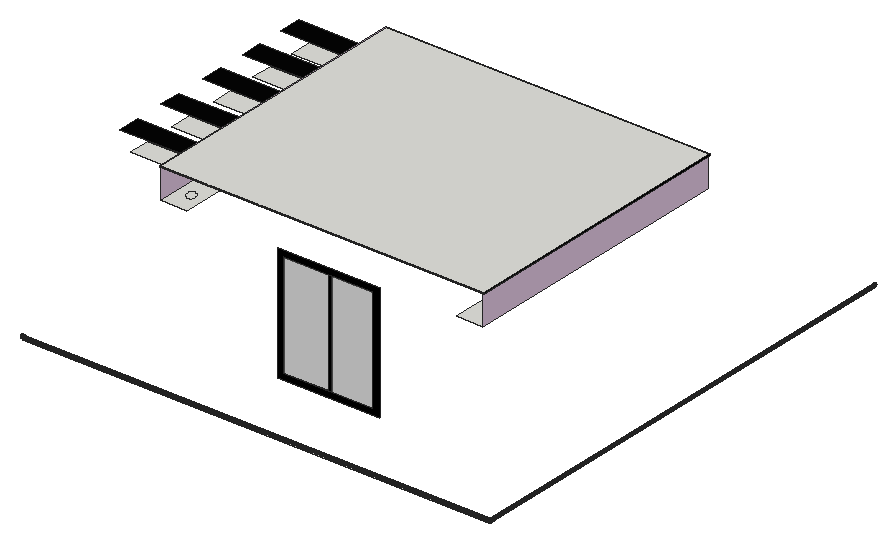
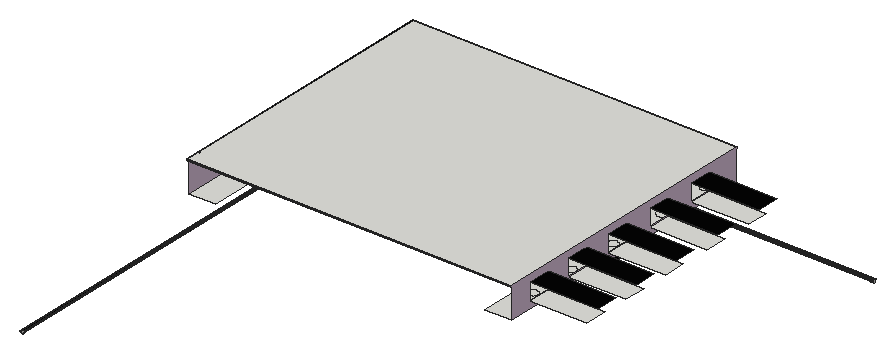
# SketchUp Ruby script. Lengths in inches.
U = 1.inch
M = Sketchup.active_model
def pt(a) = Geom::Point3d.new(a.map { |v| v * U })
def face(e, loops, mat)
  f = e.add_face(loops[0].map { |a| pt(a) })
  loops[1..].each { |l| e.add_face(l.map { |a| pt(a) }).erase! }
  f.material = f.back_material = mat if mat
  f
end
# faces: each face lists its corners as indices into pts; further lists are holes
def faces(e, pts, list, mat = nil) = list.each { |f| face(e, (f[0].is_a?(Array) ? f : [f]).map { |l| l.map { |i| pts[i] } }, mat) }
# xy, xz, yz: faces in a plane at the given z, y or x. An outline is a flat list of corners, or four numbers for a rectangle; further outlines are holes
def ring(l) = l.size == 4 ? [[l[0], l[1]], [l[2], l[1]], [l[2], l[3]], [l[0], l[3]]] : l.each_slice(2).to_a
def flat(e, list, mat, &to3) = list.each { |f| face(e, (f[0].is_a?(Array) ? f : [f]).map { |l| ring(l).map { |u, v| to3.(u, v) } }, mat) }
def xy(e, z, list, mat = nil) = flat(e, list, mat) { |x, y| [x, y, z] }
def xz(e, y, list, mat = nil) = flat(e, list, mat) { |x, z| [x, y, z] }
def yz(e, x, list, mat = nil) = flat(e, list, mat) { |y, z| [x, y, z] }
def lines(e, pts, list) = list.each { |a, b| e.add_line(pt(pts[a]), pt(pts[b])) }
# prism: a flat outline (further loops are holes) pulled along v
def prism(e, loops, v, mat = nil)
  f = face(e, loops, mat); d = Geom::Vector3d.new(v.map { |x| x * U })
  f.pushpull(f.normal.samedirection?(d) ? d.length : -d.length)
end
def box(e, o, s, mat = nil) = prism(e, [[o, [o[0] + s[0], o[1], o[2]], [o[0] + s[0], o[1] + s[1], o[2]], [o[0], o[1] + s[1], o[2]]]], [0, 0, s[2]], mat)
def at(x, y, z, deg = 0) = Geom::Transformation.translation(pt([x, y, z])) * Geom::Transformation.rotation(ORIGIN, Z_AXIS, deg.degrees)
def axes(o, x, y, z) = Geom::Transformation.new([*x, 0, *y, 0, *z, 0, *pt(o).to_a, 1])
def part(name) = M.definitions.add(name)
# library, detail: a bought-in or finely detailed component or shape, given as its bounding box
def library(name, o, s) = part(name).tap { |d| box(d.entities, o, s) }
def detail(e, o, s) = box(e.add_group.entities, o, s)
def put(e, d, t, mat = nil) = e.add_instance(d, t).tap { |i| i.material = mat if mat }
def group(e, t, mat = nil) = e.add_group.tap { |g| g.transformation = t; g.material = mat if mat }.entities
root = M.entities
M.materials.add("[0118_Thistle]").color = [216, 191, 216]
M.materials.add("[0136_Charcoal]").color = [5, 5, 5]
M.materials.add("[0137_Black]").color = [0, 0, 0]
M.materials.add("[Translucent Glass Gray]").color = [128, 128, 128]
M.materials["[Translucent Glass Gray]"].alpha = 0.5
xy(root,1352.375,[[8.99,75.58,1077.01,78.58]])
xy(root,1354.0625,[[1079.8,75.38,1080.11,75.38,1080.42,75.4,1080.73,75.47,1081.03,75.56,1081.32,75.68,1081.59,75.83,1081.85,76.01,1082.09,76.22,1082.3,76.45,1082.49,76.7,1082.65,76.97,1082.78,77.26,1082.89,77.55,1082.96,77.86,1082.99,78.17,1083,78.48,1082.97,78.8,1082.91,79.11,1082.82,79.41,1082.69,79.69,1082.54,79.97,1082.36,80.23,1082.15,80.46,1081.92,80.68,1081.67,80.86,1081.4,81.03,1081.12,81.16,1080.82,81.26,1080.52,81.33,1080.2,81.37,1079.89,81.37,1079.58,81.35,1079.27,81.28,1078.97,81.19,1078.68,81.07,1078.41,80.92,1078.15,80.74,1077.91,80.53,1077.7,80.3,1077.51,80.05,1077.35,79.78,1077.22,79.49,1077.11,79.2,1077.04,78.89,1077.01,78.58,1077,78.375,1077,78.27,1077.03,77.95,1077.09,77.64,1077.18,77.34,1077.31,77.06,1077.46,76.78,1077.64,76.52,1077.85,76.29,1078.08,76.07,1078.33,75.89,1078.6,75.72,1078.88,75.59,1079.18,75.49,1079.48,75.42]])
xy(root,1354.07,[[1079.86,81.375,1080.18,1173.38]],"[0137_Black]")
xy(root,1360.06,[[1079.82,81.375,1080.14,1179.37]],"[0137_Black]")
xy(root,1597.0625,[[[156,288.375,216,930.375],[186.49,446.54,189.62,446.78,192.57,447.82,195.16,449.58,197.2,451.96,198.55,454.78,199.13,457.86,198.9,460.99,197.86,463.94,196.09,466.53,193.72,468.57,190.89,469.93,187.8125,470.5,184.6875,470.27,181.73,469.23,179.15,467.46,177.11,465.09,175.75,462.26,175.17,459.18,175.41,456.06,176.45,453.1,178.21,450.52,180.59,448.48,183.41,447.12],[186.49,587.35,189.62,587.59,192.57,588.63,195.16,590.4,197.2,592.77,198.55,595.6,199.13,598.68,198.9,601.8,197.86,604.75,196.09,607.34,193.72,609.38,190.89,610.74,187.8125,611.32,184.6875,611.08,181.73,610.04,179.15,608.28,177.11,605.9,175.75,603.07,175.17,600,175.41,596.87,176.45,593.92,178.21,591.33,180.59,589.29,183.41,587.93],[186.49,708.35,189.62,708.59,192.57,709.63,195.16,711.4,197.2,713.77,198.55,716.6,199.13,719.68,198.9,722.8,197.86,725.75,196.09,728.34,193.72,730.38,190.89,731.74,187.8125,732.32,184.6875,732.08,181.73,731.04,179.15,729.28,177.11,726.9,175.75,724.07,175.17,721,175.41,717.87,176.45,714.92,178.21,712.33,180.59,710.29,183.41,708.93],[186.49,324.85,189.62,325.09,192.57,326.13,195.16,327.9,197.2,330.27,198.55,333.1,199.13,336.18,198.9,339.3,197.86,342.25,196.09,344.84,193.72,346.88,190.89,348.24,187.8125,348.82,184.6875,348.58,181.73,347.54,179.15,345.78,177.11,343.4,175.75,340.57,175.17,337.5,175.41,334.37,176.45,331.42,178.21,328.83,180.59,326.79,183.41,325.43],[186.49,817.29,189.62,817.53,192.57,818.57,195.16,820.33,197.2,822.71,198.55,825.53,199.13,828.61,198.9,831.74,197.86,834.69,196.09,837.28,193.72,839.32,190.89,840.68,187.8125,841.25,184.6875,841.02,181.73,839.98,179.15,838.21,177.11,835.84,175.75,833.01,175.17,829.93,175.41,826.81,176.45,823.85,178.21,821.27,180.59,819.23,183.41,817.87]],[834,288.375,894,930.375],[186.49,324.85,183.41,325.43,180.59,326.79,178.21,328.83,176.45,331.42,175.41,334.37,175.17,337.5,175.75,340.57,177.11,343.4,179.15,345.78,181.73,347.54,184.6875,348.58,187.8125,348.82,190.89,348.24,193.72,346.88,196.09,344.84,197.86,342.25,198.9,339.3,199.13,336.18,198.55,333.1,197.2,330.27,195.16,327.9,192.57,326.13,189.62,325.09],[186.49,446.54,183.41,447.12,180.59,448.48,178.21,450.52,176.45,453.1,175.41,456.06,175.17,459.18,175.75,462.26,177.11,465.09,179.15,467.46,181.73,469.23,184.6875,470.27,187.8125,470.5,190.89,469.93,193.72,468.57,196.09,466.53,197.86,463.94,198.9,460.99,199.13,457.86,198.55,454.78,197.2,451.96,195.16,449.58,192.57,447.82,189.62,446.78],[186.49,587.35,183.41,587.93,180.59,589.29,178.21,591.33,176.45,593.92,175.41,596.87,175.17,600,175.75,603.07,177.11,605.9,179.15,608.28,181.73,610.04,184.6875,611.08,187.8125,611.32,190.89,610.74,193.72,609.38,196.09,607.34,197.86,604.75,198.9,601.8,199.13,598.68,198.55,595.6,197.2,592.77,195.16,590.4,192.57,588.63,189.62,587.59],
  [186.49,708.35,183.41,708.93,180.59,710.29,178.21,712.33,176.45,714.92,175.41,717.87,175.17,721,175.75,724.07,177.11,726.9,179.15,729.28,181.73,731.04,184.6875,732.08,187.8125,732.32,190.89,731.74,193.72,730.38,196.09,728.34,197.86,725.75,198.9,722.8,199.13,719.68,198.55,716.6,197.2,713.77,195.16,711.4,192.57,709.63,189.62,708.59],[186.49,817.29,183.41,817.87,180.59,819.23,178.21,821.27,176.45,823.85,175.41,826.81,175.17,829.93,175.75,833.01,177.11,835.84,179.15,838.21,181.73,839.98,184.6875,841.02,187.8125,841.25,190.89,840.68,193.72,839.32,196.09,837.28,197.86,834.69,198.9,831.74,199.13,828.61,198.55,825.53,197.2,822.71,195.16,820.33,192.57,818.57,189.62,817.53]])
xy(root,1614.61,[[24.25,366.56,156,417.12],[24.25,484.62,156,535.18],[24.25,604.12,156,654.68],[24.25,717.12,156,767.68],[24.25,827.68,156,878.24]])
xy(root,1652.92,[[0,366.56,156,417.12],[0,484.62,156,535.18],[0,604.12,156,654.68],[0,717.12,156,767.68],[0,827.68,156,878.24]],"[0136_Charcoal]")
xy(root,1666.0625,[[156,285.375,897,288.375],[894,288.375,897,933.375],[156,930.375,894,933.375]])
xy(root,1669.0625,[[156,285.375,897,933.375]])
xz(root,81.375,[[5.97,1354.0625,6,1354.0625,6,1357.0625,9,1357.0625,8.99,1357.35,8.94,1357.66,8.86,1357.97,8.75,1358.26,8.61,1358.54,8.44,1358.81,8.25,1359.05,8.03,1359.28,7.78,1359.47,7.52,1359.65,7.24,1359.79,6.95,1359.91,6.65,1359.99,6.34,1360.04,6.03,1360.0625,5.71,1360.05,5.4,1360,5.1,1359.92,4.8,1359.8125,4.52,1359.67,4.26,1359.5,4.01,1359.31,3.79,1359.09,3.59,1358.85,3.41,1358.58,3.27,1358.31,3.15,1358.01,3.07,1357.71,3.02,1357.4,3,1357.09,3.01,1356.77,3.06,1356.46,3.14,1356.16,3.25,1355.87,3.39,1355.58,3.56,1355.32,3.75,1355.07,3.97,1354.85,4.22,1354.65,4.48,1354.48,4.76,1354.33,5.05,1354.22,5.35,1354.13,5.66,1354.08],[6,1354.0625,6.29,1354.08,6.6,1354.12,6.9,1354.2,7.2,1354.3125,7.48,1354.45,7.74,1354.62,7.99,1354.82,8.21,1355.04,8.41,1355.28,8.59,1355.54,8.73,1355.82,8.85,1356.11,8.93,1356.41,8.98,1356.72,9,1357.04,9,1357.0625,6,1357.0625],[1079.86,1354.07,1080.18,1354.07,1080.49,1354.1,1080.79,1354.17,1081.09,1354.27,1081.38,1354.4,1081.65,1354.56,1081.9,1354.74,1082.13,1354.95,1082.34,1355.1875,1082.53,1355.44,1082.68,1355.72,1082.81,1356,1082.9,1356.3,1082.97,1356.61,1083,1356.92,1082.99,1357.24,1082.96,1357.55,1082.89,1357.86,1082.79,1358.15,1082.66,1358.44,1082.51,1358.71,1082.32,1358.96,1082.11,1359.2,1081.875,1359.41,1081.62,1359.59,1081.35,1359.74,1081.06,1359.87,1080.76,1359.96,1080.45,1360.03,1080.14,1360.06,1079.82,1360.06,1079.51,1360.02,1079.21,1359.96,1078.91,1359.86,1078.62,1359.73,1078.35,1359.57,1078.1,1359.38,1077.87,1359.17,1077.66,1358.9375,1077.47,1358.68,1077.32,1358.41,1077.19,1358.12,1077.1,1357.82,1077.03,1357.51,1077,1357.2,1077,1357.0625,1077.01,1356.89,1077.04,1356.57,1077.11,1356.27,1077.21,1355.97,1077.34,1355.68,1077.49,1355.41,1077.68,1355.16,1077.89,1354.93,1078.125,1354.72,1078.38,1354.54,1078.65,1354.38,1078.94,1354.26,1079.24,1354.16,1079.55,1354.1]])
xz(root,285.375,[[156,1666.0625,897,1669.0625]],"[0137_Black]")
xz(root,288.375,[[[423.26,1325.51,656.88,1594.07],[437.95,1340.2,642.2,1579.38]],[540.07,1340.2,547.42,1579.38]],"[0137_Black]")
xz(root,288.375,[[437.95,1340.2,540.07,1579.38],[547.42,1340.2,642.2,1579.38]],"[Translucent Glass Gray]")
xz(root,933.375,[[156,1666.0625,897,1669.0625]],"[0137_Black]")
yz(root,156,[[[288.375,1597.0625,288.375,1666.0625,285.375,1666.0625,285.375,1669.0625,933.375,1669.0625,933.375,1666.0625,930.375,1666.0625,930.375,1597.0625],[827.68,1614.61,878.24,1652.92],[717.12,1614.61,767.68,1652.92],[604.12,1614.61,654.68,1652.92],[484.62,1614.61,535.18,1652.92],[366.56,1614.61,417.12,1652.92]]],"[0118_Thistle]")
yz(root,894,[[288.375,1597.0625,930.375,1666.0625]],"[0118_Thistle]")
yz(root,897,[[285.375,1666.0625,933.375,1669.0625]],"[0137_Black]")
p = [[8.85,77.45,1354.21],[8.93,77.75,1354.13],[1080,77.75,1354.13],[1080,77.45,1354.21],[8.98,78.0625,1354.08],[1080,78.0625,1354.08],
  [9,78.375,1354.0625],[1077,78.375,1354.0625],[1080,78.375,1354.0625],[8.98,78.6875,1354.08],[1080,78.6875,1354.08],[8.93,79,1354.13],
  [1080,79,1354.13],[8.85,79.3,1354.21],[1080,79.3,1354.21],[1079.24,1173.47,1354.16],[1079.55,1173.41,1354.1],[1079.55,81.375,1354.1],
  [1079.24,81.375,1354.16],[1079.86,1173.38,1354.07],[1079.86,81.375,1354.07],[1080.18,1173.38,1354.07],[1080.49,1173.41,1354.1],[1080.49,81.375,1354.1],
  [1080.18,81.375,1354.07],[1080.79,1173.48,1354.17],[1080.79,81.375,1354.17],[1077.01,1176.2,1354.09],[1077.01,1175.79,1354.12],[1077.01,1175.05,1354.37],
  [1077.02,1174.4,1354.81],[1077.02,1173.88,1355.4],[1077.02,1173.53,1356.1],[1077.02,1173.38,1356.87],[1077.02,1173.43,1357.65],[1077.02,1173.69,1358.39],
  [1077.02,1174.12,1359.04],[1077.01,1174.71,1359.56],[1077.01,1175.41,1359.9],[1077.01,1176.18,1360.06],[1077,1176.96,1360],[1077,1177.7,1359.75],
  [1076.99,1178.35,1359.32],[1076.99,1178.87,1358.73],[1076.99,1179.22,1358.03],[1076.99,1179.37,1357.26],[1076.99,1179.32,1356.48],[1076.99,1179.06,1355.73],
  [1076.99,1178.63,1355.08],[1076.99,1178.04,1354.57],[1077,1177.34,1354.22],[1077,1176.57,1354.07],[1077,1176.51,1354.07],[1077,1176.51,1357.2],
  [1077,1176.375,1357.0625],[1077.01,1176.2,1356.89],[8.74,77.15,1354.32],[1080,77.15,1354.32],[8.74,79.6,1354.32],[1080,79.6,1354.32],
  [1078.94,1173.57,1354.26],[1078.94,81.375,1354.26],[1081.09,1173.58,1354.27],[1081.09,81.375,1354.27],[8.6,76.875,1354.46],[1080,76.875,1354.46],
  [8.6,79.875,1354.46],[1080,79.875,1354.46],[1078.65,1173.69,1354.38],[1078.65,81.375,1354.38],[1081.38,1173.71,1354.4],[1081.38,81.375,1354.4],
  [1078.38,1173.85,1354.54],[1078.38,81.375,1354.54],[1081.65,1173.87,1354.56],[1081.65,81.375,1354.56],[8.43,76.61,1354.64],[1080,76.61,1354.64],
  [8.43,80.14,1354.64],[1080,80.14,1354.64],[1078.125,1174.03,1354.72],[1078.125,81.375,1354.72],[8.23,76.37,1354.83],[1080,76.37,1354.83],
  [8.23,80.38,1354.83],[1080,80.38,1354.83],[1081.9,1174.06,1354.74],[1081.9,81.375,1354.74],[1077.89,1174.24,1354.93],[1077.89,81.375,1354.93],
  [1082.13,1174.27,1354.95],[1082.13,81.375,1354.95],[8.01,76.15,1355.06],[1080,76.15,1355.06],[8.01,80.6,1355.06],[1080,80.6,1355.06],
  [1077.68,1174.47,1355.16],[1077.68,81.375,1355.16],[1082.34,1174.5,1355.1875],[1082.34,81.375,1355.1875],[7.76,75.95,1355.3],[1080,75.95,1355.3],
  [7.76,80.8,1355.3],[1080,80.8,1355.3],[1077.49,1174.73,1355.41],[1077.49,81.375,1355.41],[1082.53,1174.76,1355.44],[1082.53,81.375,1355.44],
  [7.5,75.78,1355.5625],[1080,75.78,1355.5625],[7.5,80.97,1355.5625],[1080,80.97,1355.5625],[1077.34,1175,1355.68],[1077.34,81.375,1355.68],
  [1082.68,1175.03,1355.72],[1082.68,81.375,1355.72],[7.22,75.63,1355.84],[1080,75.63,1355.84],[7.22,81.12,1355.84],[1080,81.12,1355.84],
  [1077.21,1175.28,1355.97],[1077.21,81.375,1355.97],[1082.81,1175.32,1356],[1082.81,81.375,1356],[6.93,75.52,1356.14],[1080,75.52,1356.14],
  [6.93,81.23,1356.14],[1080,81.23,1356.14],[1077.11,1175.58,1356.27],[1077.11,81.375,1356.27],[1082.9,1175.62,1356.3],[1082.9,81.375,1356.3],
  [6.625,75.44,1356.4375],[1080,75.44,1356.4375],[6.625,81.31,1356.4375],[1080,81.31,1356.4375],[1077.04,1175.89,1356.57],[1077.04,81.375,1356.57],
  [1082.97,1175.92,1356.61],[1082.97,81.375,1356.61],[6.3125,75.39,1356.75],[1080,75.39,1356.75],[6.3125,81.36,1356.75],[1080,81.36,1356.75],
  [1077.01,81.375,1356.89],[1083,1176.24,1356.92],[1083,81.375,1356.92],[6,75.375,1357.0625],[1080,75.375,1357.0625],[6,81.375,1357.0625],
  [9,81.375,1357.0625],[1077,81.375,1357.0625],[1080,81.375,1357.0625],[1077,81.375,1357.2],[1082.99,1176.55,1357.24],[1082.99,81.375,1357.24],
  [5.6875,75.39,1357.375],[1080,75.39,1357.375],[5.6875,81.36,1357.375],[1080,81.36,1357.375],[1077.03,1176.83,1357.51],[1077.03,81.375,1357.51],
  [1082.96,1176.86,1357.55],[1082.96,81.375,1357.55],[5.375,75.44,1357.6875],[1080,75.44,1357.6875],[5.375,81.31,1357.6875],[1080,81.31,1357.6875],
  [1077.1,1177.13,1357.82],[1077.1,81.375,1357.82],[1082.89,1177.17,1357.86],[1082.89,81.375,1357.86],[5.07,75.52,1357.99],[1080,75.52,1357.99],
  [5.07,81.23,1357.99],[1080,81.23,1357.99],[1077.19,1177.43,1358.12],[1077.19,81.375,1358.12],[1082.79,1177.47,1358.15],[1082.79,81.375,1358.15],
  [4.78,75.63,1358.28],[1080,75.63,1358.28],[4.78,81.12,1358.28],[1080,81.12,1358.28],[1077.32,1177.72,1358.41],[1077.32,81.375,1358.41],
  [1082.66,1177.75,1358.44],[1082.66,81.375,1358.44],[4.5,75.78,1358.5625],[1080,75.78,1358.5625],[4.5,80.97,1358.5625],[1080,80.97,1358.5625],
  [1077.47,1177.99,1358.68],[1077.47,81.375,1358.68],[1082.51,1178.02,1358.71],[1082.51,81.375,1358.71],[4.24,75.95,1358.83],[1080,75.95,1358.83],
  [4.24,80.8,1358.83],[1080,80.8,1358.83],[1077.66,1178.25,1358.9375],[1077.66,81.375,1358.9375],[1082.32,1178.28,1358.96],[1082.32,81.375,1358.96],
  [3.99,76.15,1359.07],[1080,76.15,1359.07],[3.99,80.6,1359.07],[1080,80.6,1359.07],[1077.87,1178.48,1359.17],[1077.87,81.375,1359.17],
  [1082.11,1178.51,1359.2],[1082.11,81.375,1359.2],[3.77,76.37,1359.29],[1080,76.37,1359.29],[3.77,80.38,1359.29],[1080,80.38,1359.29],
  [1078.1,1178.69,1359.38],[1078.1,81.375,1359.38],[1081.875,1178.72,1359.41],[1081.875,81.375,1359.41],[3.57,76.61,1359.49],[1080,76.61,1359.49],
  [3.57,80.14,1359.49],[1080,80.14,1359.49],[1078.35,1178.88,1359.57],[1078.35,81.375,1359.57],[1081.62,1178.9,1359.59],[1081.62,81.375,1359.59],
  [3.4,76.875,1359.66],[1080,76.875,1359.66],[3.4,79.875,1359.66],[1080,79.875,1359.66],[1078.62,1179.04,1359.73],[1078.62,81.375,1359.73],
  [1081.35,1179.06,1359.74],[1081.35,81.375,1359.74],[3.26,77.15,1359.8],[1080,77.15,1359.8],[3.26,79.6,1359.8],[1080,79.6,1359.8],
  [1078.91,1179.17,1359.86],[1078.91,81.375,1359.86],[1081.06,1179.18,1359.87],[1081.06,81.375,1359.87],[3.15,77.45,1359.92],[1080,77.45,1359.92],
  [3.15,79.3,1359.92],[1080,79.3,1359.92],[3.07,77.75,1360],[1080,77.75,1360],[3.07,79,1360],[1080,79,1360],
  [1079.21,1179.27,1359.96],[1079.21,81.375,1359.96],[1080.76,1179.28,1359.96],[1080.76,81.375,1359.96],[3.02,78.0625,1360.05],[1080,78.0625,1360.05],
  [3,78.375,1360.0625],[1080,78.375,1360.0625],[3.02,78.6875,1360.05],[1080,78.6875,1360.05],[1079.51,1179.34,1360.02],[1079.51,81.375,1360.02],
  [1079.82,1179.37,1360.06],[1079.82,81.375,1360.06],[1080.45,1179.34,1360.03],[1080.14,1179.37,1360.06],[1080.14,81.375,1360.06],[1080.45,81.375,1360.03],
  [6,78.375,1357.0625],[1080,78.375,1357.0625],[1080,1176.375,1357.0625]]
faces(root,p,[[0,1,2,3],[4,6,7,8,5],[6,9,10,8,7],[9,11,12,10],[11,13,14,12],[27,28,29,30,31,32,33,34,35,36,37,38,39,40,41,42,43,44,45,46,47,48,49,50,51,52,53,54,55],[53,52,27,55,54],[13,58,59,14],
  [58,66,67,59],[66,78,79,67],[78,84,85,79],[84,94,95,85],[94,102,103,95],[102,110,111,103],[110,118,119,111],[118,126,127,119],
  [126,134,135,127],[134,142,143,135],[142,149,150,151,152,143],[149,158,159,152,151,150],[158,166,167,159],[166,174,175,167],[174,182,183,175],[182,190,191,183],
  [190,198,199,191],[198,206,207,199],[206,214,215,207],[214,222,223,215],[222,230,231,223],[230,238,239,231],[244,236,237,245],[238,246,247,239],
  [248,244,245,249],[246,250,251,247],[256,248,249,257],[258,256,257,259],[260,258,259,261],[250,260,261,251]])
faces(root,p,[[1,4,5,2],[15,16,17,18],[16,19,20,17],[21,22,23,24],[22,25,26,23],[56,0,3,57],[60,15,18,61],[25,62,63,26],
  [64,56,57,65],[68,60,61,69],[62,70,71,63],[72,68,69,73],[70,74,75,71],[76,64,65,77],[80,72,73,81],[82,76,77,83],
  [74,86,87,75],[88,80,81,89],[86,90,91,87],[92,82,83,93],[96,88,89,97],[90,98,99,91],[100,92,93,101],[104,96,97,105],
  [98,106,107,99],[108,100,101,109],[112,104,105,113],[106,114,115,107],[116,108,109,117],[120,112,113,121],[114,122,123,115],[124,116,117,125],
  [128,120,121,129],[122,130,131,123],[132,124,125,133],[136,128,129,137],[130,138,139,131],[140,132,133,141],[55,136,137,144],[138,145,146,139],
  [147,140,141,148],[54,55,144,151,153,53],[145,154,155,146],[156,147,148,157],[160,53,153,161],[154,162,163,155],[164,156,157,165],[168,160,161,169],
  [162,170,171,163],[172,164,165,173],[176,168,169,177],[170,178,179,171],[180,172,173,181],[184,176,177,185],[178,186,187,179],[188,180,181,189],
  [192,184,185,193],[186,194,195,187],[196,188,189,197],[200,192,193,201],[194,202,203,195],[204,196,197,205],[208,200,201,209],[202,210,211,203],
  [212,204,205,213],[216,208,209,217],[210,218,219,211],[220,212,213,221],[224,216,217,225],[218,226,227,219],[228,220,221,229],[232,224,225,233],
  [226,234,235,227],[236,228,229,237],[240,232,233,241],[234,242,243,235],[252,240,241,253],[242,254,255,243],[262,252,253,263],[264,262,263,265],
  [266,267,268,269],[254,266,269,255]],"[0137_Black]")
lines(root,p,[[270,271],[272,54],[152,272]])
